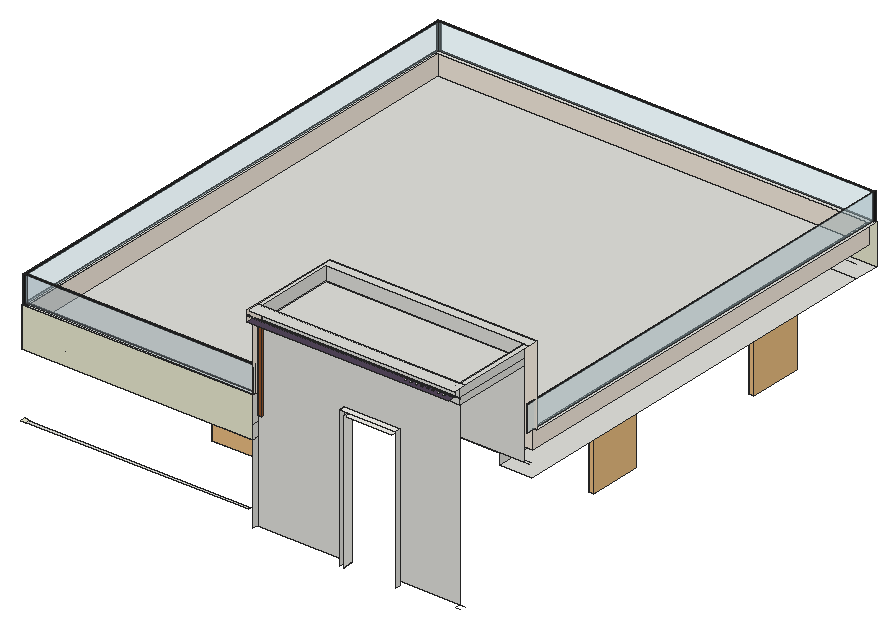
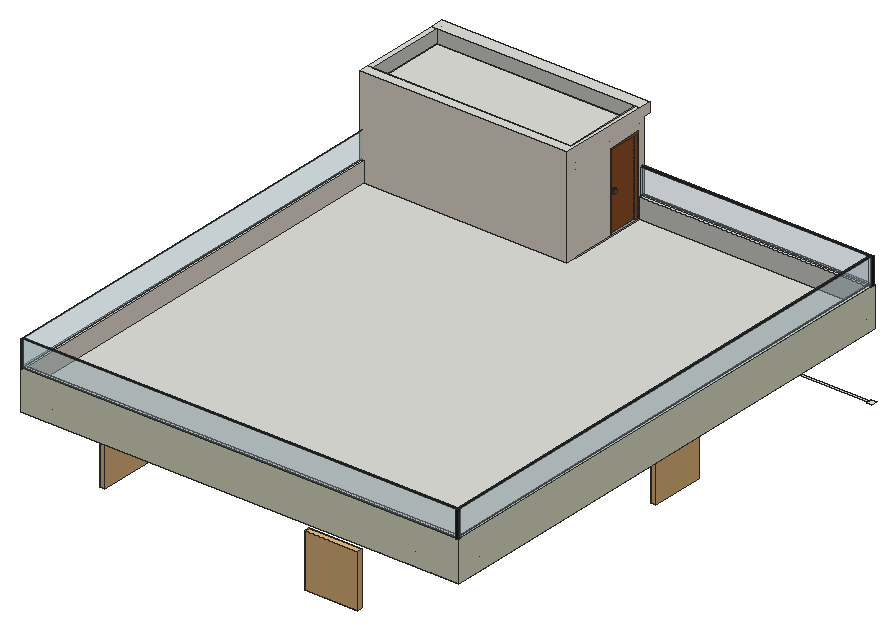
# SketchUp Ruby script. Lengths in inches.
U = 1.inch
M = Sketchup.active_model
def pt(a) = Geom::Point3d.new(a.map { |v| v * U })
def face(e, loops, mat)
  f = e.add_face(loops[0].map { |a| pt(a) })
  loops[1..].each { |l| e.add_face(l.map { |a| pt(a) }).erase! }
  f.material = f.back_material = mat if mat
  f
end
# faces: each face lists its corners as indices into pts; further lists are holes
def faces(e, pts, list, mat = nil) = list.each { |f| face(e, (f[0].is_a?(Array) ? f : [f]).map { |l| l.map { |i| pts[i] } }, mat) }
# xy, xz, yz: faces in a plane at the given z, y or x. An outline is a flat list of corners, or four numbers for a rectangle; further outlines are holes
def ring(l) = l.size == 4 ? [[l[0], l[1]], [l[2], l[1]], [l[2], l[3]], [l[0], l[3]]] : l.each_slice(2).to_a
def flat(e, list, mat, &to3) = list.each { |f| face(e, (f[0].is_a?(Array) ? f : [f]).map { |l| ring(l).map { |u, v| to3.(u, v) } }, mat) }
def xy(e, z, list, mat = nil) = flat(e, list, mat) { |x, y| [x, y, z] }
def xz(e, y, list, mat = nil) = flat(e, list, mat) { |x, z| [x, y, z] }
def yz(e, x, list, mat = nil) = flat(e, list, mat) { |y, z| [x, y, z] }
def lines(e, pts, list) = list.each { |a, b| e.add_line(pt(pts[a]), pt(pts[b])) }
# prism: a flat outline (further loops are holes) pulled along v
def prism(e, loops, v, mat = nil)
  f = face(e, loops, mat); d = Geom::Vector3d.new(v.map { |x| x * U })
  f.pushpull(f.normal.samedirection?(d) ? d.length : -d.length)
end
def box(e, o, s, mat = nil) = prism(e, [[o, [o[0] + s[0], o[1], o[2]], [o[0] + s[0], o[1] + s[1], o[2]], [o[0], o[1] + s[1], o[2]]]], [0, 0, s[2]], mat)
def at(x, y, z, deg = 0) = Geom::Transformation.translation(pt([x, y, z])) * Geom::Transformation.rotation(ORIGIN, Z_AXIS, deg.degrees)
def axes(o, x, y, z) = Geom::Transformation.new([*x, 0, *y, 0, *z, 0, *pt(o).to_a, 1])
def part(name) = M.definitions.add(name)
# library, detail: a bought-in or finely detailed component or shape, given as its bounding box
def library(name, o, s) = part(name).tap { |d| box(d.entities, o, s) }
def detail(e, o, s) = box(e.add_group.entities, o, s)
def put(e, d, t, mat = nil) = e.add_instance(d, t).tap { |i| i.material = mat if mat }
def group(e, t, mat = nil) = e.add_group.tap { |g| g.transformation = t; g.material = mat if mat }.entities
root = M.entities
M.materials.add("0037 AP 8028 PEACH ORGANZA").color = [246, 236, 223]
M.materials.add("0113 AP L161 ABSOLUTE WHITE").color = [243, 242, 236]
M.materials.add("0280 AP 9627 Emperor_s Purple-N").color = [83, 70, 91]
M.materials.add("0746 AP 7715 LUMINOUS").color = [235, 235, 209]
M.materials.add("Glass_Basic_01").color = [161, 173, 186]
M.materials["Glass_Basic_01"].alpha = 0.25
M.materials.add("Glass_Safety_01").color = [204, 235, 244]
M.materials["Glass_Safety_01"].alpha = 0.25
M.materials.add("M08_Obsidian_Black").color = [30, 30, 30]
M.materials.add("[Color M00]").color = [255, 255, 255]
M.materials.add("[Color M08]").color = [30, 30, 30]
M.materials.add("[Wood_Cherry_Original]").color = [152, 86, 42]
M.materials.add("[Wood_Lumber_ButtJoined]").color = [164, 152, 112]
c1 = library("Slide Window 5'",[0,-2.02,0],[60,2.02,54])
c2 = part("Electrical junction box")
xy(c2.entities,0,[[0.77,1.5,0.75,1.502,0.64,1.512,0.518,1.557,0.411,1.632,0.328,1.733,0.273,1.851,0.25,1.98,0.262,2.11,0.307,2.232,0.382,2.339,0.483,2.422,0.601,2.477,0.73,2.5,0.75,2.498,0.86,2.488,0.982,2.443,1.089,2.368,1.172,2.267,1.227,2.149,1.25,2.02,1.238,1.89,1.193,1.768,1.118,1.661,1.017,1.578,0.899,1.523]],"[Color M00]")
xy(c2.entities,0,[[[0,0,1.5,4],[0.77,1.5,0.899,1.523,1.017,1.578,1.118,1.661,1.193,1.768,1.238,1.89,1.25,2.02,1.227,2.149,1.172,2.267,1.089,2.368,0.982,2.443,0.86,2.488,0.75,2.498,0.73,2.5,0.601,2.477,0.483,2.422,0.382,2.339,0.307,2.232,0.262,2.11,0.25,1.98,0.273,1.851,0.328,1.733,0.411,1.632,0.518,1.557,0.64,1.512,0.75,1.502]]],"[Color M08]")
xy(c2.entities,4,[[0.75,1.502,0.879,1.525,0.997,1.579,1.097,1.663,1.172,1.77,1.217,1.892,1.229,2.022,1.207,2.151,1.152,2.269,1.068,2.37,0.962,2.445,0.839,2.49,0.75,2.498,0.73,2.5,0.709,2.501,0.581,2.479,0.462,2.424,0.362,2.341,0.287,2.234,0.242,2.111,0.23,1.981,0.252,1.853,0.307,1.734,0.391,1.634,0.497,1.559,0.62,1.514,0.73,1.504]],"[Color M00]")
xy(c2.entities,4,[[[0,0,1.5,4],[0.75,1.502,0.73,1.504,0.62,1.514,0.497,1.559,0.391,1.634,0.307,1.734,0.252,1.853,0.23,1.981,0.242,2.111,0.287,2.234,0.362,2.341,0.462,2.424,0.581,2.479,0.709,2.501,0.73,2.5,0.75,2.498,0.839,2.49,0.962,2.445,1.068,2.37,1.152,2.269,1.207,2.151,1.229,2.022,1.217,1.892,1.172,1.77,1.097,1.663,0.997,1.579,0.879,1.525]]],"[Color M08]")
xz(c2.entities,0,[[0.77,1.5,0.899,1.523,1.017,1.578,1.118,1.661,1.193,1.768,1.238,1.89,1.25,2.02,1.227,2.149,1.172,2.267,1.089,2.368,0.982,2.443,0.86,2.488,0.75,2.498,0.73,2.5,0.601,2.477,0.483,2.422,0.382,2.339,0.307,2.232,0.262,2.11,0.25,1.98,0.273,1.851,0.328,1.733,0.411,1.632,0.518,1.557,0.64,1.512,0.75,1.502]],"[Color M00]")
xz(c2.entities,0,[[[0,0,1.5,4],[0.77,1.5,0.75,1.502,0.64,1.512,0.518,1.557,0.411,1.632,0.328,1.733,0.273,1.851,0.25,1.98,0.262,2.11,0.307,2.232,0.382,2.339,0.483,2.422,0.601,2.477,0.73,2.5,0.75,2.498,0.86,2.488,0.982,2.443,1.089,2.368,1.172,2.267,1.227,2.149,1.25,2.02,1.238,1.89,1.193,1.768,1.118,1.661,1.017,1.578,0.899,1.523]]],"[Color M08]")
xz(c2.entities,4,[[0.73,1.5,0.601,1.523,0.483,1.578,0.382,1.661,0.307,1.768,0.262,1.89,0.25,2.02,0.273,2.149,0.328,2.267,0.411,2.368,0.518,2.443,0.64,2.488,0.75,2.498,0.77,2.5,0.899,2.477,1.017,2.422,1.118,2.339,1.193,2.232,1.238,2.11,1.25,1.98,1.227,1.851,1.172,1.733,1.089,1.632,0.982,1.557,0.86,1.512,0.75,1.502]],"[Color M00]")
xz(c2.entities,4,[[[0,0,1.5,4],[0.73,1.5,0.75,1.502,0.86,1.512,0.982,1.557,1.089,1.632,1.172,1.733,1.227,1.851,1.25,1.98,1.238,2.11,1.193,2.232,1.118,2.339,1.017,2.422,0.899,2.477,0.77,2.5,0.75,2.498,0.64,2.488,0.518,2.443,0.411,2.368,0.328,2.267,0.273,2.149,0.25,2.02,0.262,1.89,0.307,1.768,0.382,1.661,0.483,1.578,0.601,1.523]]],"[Color M08]")
yz(c2.entities,0,[[0,0,4,4]],"[Color M08]")
yz(c2.entities,1.5,[[0,0,4,4]],"[Color M08]")
p = [[0.75,2.498,4],[0.75,2.502,4]]
lines(c2.entities,p,[[0,1]])
c3 = library("Group\#25",[0,-0.05,0],[30,2.55,24])
xy(root,164.58,[[2160.9,113.67,2361.69,115.67]])
xy(root,164.58,[[2155.9,112.36,2160.9,117.37]],"0746 AP 7715 LUMINOUS")
xy(root,199.5,[[2205.9,189.89,2253.93,198.88],[2427.9,198.88,2432.9,228.89],[2196.91,383.38,2205.9,431.37],[2427.9,383.38,2432.9,413.39]])
xy(root,223.5,[[2157.2,112.36,2196.91,121.52],[2196.91,112.36,2366.69,121.52],[2157.2,121.52,2196.91,560.39],[2525.88,192.78,2554.91,560.39],[2157.2,560.39,2196.91,583.09],
  [2196.91,560.39,2525.88,583.09],[2525.88,560.39,2554.91,583.09]])
xy(root,235.5,[[[2196.91,121.52,2366.69,121.52,2366.69,189.89,2525.88,189.89,2525.88,560.39,2196.91,560.39,2196.91,431.37,2205.9,431.37,2205.9,383.38,2196.91,383.38],[2205.9,189.89,2253.93,198.88],[2427.9,383.38,2432.9,413.39],[2427.9,198.88,2432.9,228.89]],[2205.9,189.89,2253.93,198.88],[2427.9,198.88,2432.9,228.89],[2196.91,383.38,2205.9,431.37],[2427.9,383.38,2432.9,413.39]])
xy(root,240,[[2196.98,190.05,2525.95,560.55]])
xy(root,241.5,[[2161.2,117.37,2366.69,117.37,2366.69,198.89,2550.91,198.89,2550.91,579.09,2161.2,579.09],[2369.92,118.67,2371.21,149.31],[2366.69,150.93,2370.69,189.89]])
xy(root,241.5,[[2366.93,117.05,2366.93,119.07,2369.92,119.07,2369.92,118.67,2371.21,118.67,2371.21,117.05],[2366.93,148.91,2366.93,150.93,2371.21,150.93,2371.21,149.31,2369.92,149.31,2369.92,148.91]],"[Wood_Cherry_Original]")
xy(root,259.5,[[2157.2,112.36,2161.2,579.09],[2161.2,112.36,2366.69,117.37],[2550.91,198.89,2554.91,583.09],[2157.2,579.09,2550.91,583.09]])
xy(root,274.5,[[2452.6,108.36,2495.6,117.37]],"0113 AP L161 ABSOLUTE WHITE")
xy(root,275.5,[[2366.93,144.21,2369.92,146.17]],"[Wood_Cherry_Original]")
xy(root,276.69,[[2368.32,142.55,2368.45,142.75]],"[Wood_Lumber_ButtJoined]")
xy(root,278.26,[[2366.93,144.21,2369.92,146.17]],"[Wood_Cherry_Original]")
xy(root,278.5,[[2448.6,108.36,2499.54,112.36]],"0113 AP L161 ABSOLUTE WHITE")
xy(root,311.42,[[2366.93,119.07,2369.92,148.91]],"[Wood_Cherry_Original]")
xy(root,311.78,[[2369.92,118.67,2371.21,149.31]])
xy(root,313.5,[[2371.21,117.37,2371.21,150.93,2370.69,150.93,2370.69,189.89,2549.9,189.89,2549.9,117.37]])
xy(root,313.5,[[2366.93,117.05,2371.21,117.37],[2366.93,117.37,2370.69,150.93],[2370.69,117.37,2371.21,150.93]],"[Wood_Cherry_Original]")
xy(root,319.5,[[2370.69,117.37,2549.9,189.89]])
xy(root,322.5,[[2506.22,109.7,2507.72,110.7],[2511.22,109.7,2512.72,110.7],[2516.22,109.7,2517.72,110.7],[2521.22,109.7,2522.72,110.7],[2526.22,109.7,2527.72,110.7],
  [2531.22,109.7,2532.72,110.7],[2536.22,109.7,2537.72,110.7],[2541.22,109.7,2542.72,110.7]])
xy(root,322.5,[[[2366.69,105.36,2549.9,112.36],[2506.22,109.7,2507.72,110.7],[2511.22,109.7,2512.72,110.7],[2516.22,109.7,2517.72,110.7],[2521.22,109.7,2522.72,110.7],[2526.22,109.7,2527.72,110.7],[2531.22,109.7,2532.72,110.7],[2536.22,109.7,2537.72,110.7],[2541.22,109.7,2542.72,110.7]]],"0280 AP 9627 Emperor_s Purple-N")
xy(root,327,[[2366.69,105.16,2552.4,105.36]])
xy(root,327.8,[[2366.69,105.16,2553.2,105.36]])
xy(root,331.5,[[2366.69,105.36,2554.91,117.37],[2366.69,117.37,2370.69,117.37,2370.69,189.89,2554.91,189.89,2554.91,198.89,2366.69,198.89],[2549.9,117.37,2554.91,189.89]])
xz(root,112.36,[[2157.2,223.5,2366.69,259.5]],"0746 AP 7715 LUMINOUS")
xz(root,117.05,[[2366.93,241.5,2371.21,313.5]],"[Wood_Cherry_Original]")
xz(root,117.37,[[2366.69,151.5,2366.69,313.5,2549.9,313.5,2549.9,151.5,2495.6,151.5,2495.6,274.5,2452.6,274.5,2452.6,151.5],[2161.2,241.5,2366.69,259.5],[2370.69,313.5,2549.9,319.5],[2370.69,319.5,2549.9,331.5]])
xz(root,118.67,[[2369.92,241.5,2371.21,311.78]])
xz(root,119.07,[[2366.93,241.5,2369.92,311.42]],"[Wood_Cherry_Original]")
xz(root,121.52,[[2196.91,223.5,2366.69,235.5]])
xz(root,142.55,[[[2368.42,276.35,2368.28,276.37,2368.15,276.42,2368.04,276.5,2367.96,276.61,2367.9,276.74,2367.88,276.87,2367.9,277.01,2367.96,277.13,2368.04,277.24,2368.15,277.32,2368.28,277.375,2368.42,277.39,2368.56,277.375,2368.6875,277.32,2368.8,277.24,2368.88,277.13,2368.9375,277.01,2368.96,276.87,2368.9375,276.74,2368.88,276.61,2368.8,276.5,2368.6875,276.42,2368.56,276.37],[2368.32,276.69,2368.45,276.69,2368.45,276.9,2368.49,276.94,2368.5,276.96,2368.51,276.99,2368.5,277.02,2368.49,277.04,2368.47,277.07,2368.43,277.09,2368.4,277.1,2368.34,277.08,2368.32,277.07,2368.31,277.04,2368.29,277.02,2368.29,276.96,2368.31,276.94,2368.32,276.92]]],"[Wood_Cherry_Original]")
xz(root,142.75,[[2368.32,276.69,2368.32,276.92,2368.34,276.9,2368.37,276.89,2368.43,276.89,2368.45,276.9,2368.45,276.69],[2368.37,276.89,2368.34,276.9,2368.32,276.92,2368.31,276.94,2368.29,276.96,2368.29,277.02,2368.31,277.04,2368.32,277.07,2368.34,277.08,2368.4,277.1,2368.43,277.09,2368.47,277.07,2368.49,277.04,2368.5,277.02,2368.51,276.99,2368.5,276.96,2368.49,276.94,2368.45,276.9,2368.43,276.89]],"[Wood_Lumber_ButtJoined]")
xz(root,144.21,[[[2366.93,275.5,2369.92,278.26],[2368.42,276.35,2368.56,276.37,2368.6875,276.42,2368.8,276.5,2368.88,276.61,2368.9375,276.74,2368.96,276.87,2368.9375,277.01,2368.88,277.13,2368.8,277.24,2368.6875,277.32,2368.56,277.375,2368.42,277.39,2368.28,277.375,2368.15,277.32,2368.04,277.24,2367.96,277.13,2367.9,277.01,2367.88,276.87,2367.9,276.74,2367.96,276.61,2368.04,276.5,2368.15,276.42,2368.28,276.37]]],"[Wood_Cherry_Original]")
xz(root,146.17,[[2366.93,275.5,2369.92,278.26]],"[Wood_Cherry_Original]")
xz(root,148.91,[[2366.93,241.5,2369.92,311.42]],"[Wood_Cherry_Original]")
xz(root,149.31,[[2369.92,241.5,2371.21,311.78]])
xz(root,150.93,[[2366.93,241.5,2370.69,313.5]])
xz(root,150.93,[[2370.69,241.5,2371.21,313.5]],"[Wood_Cherry_Original]")
xz(root,189.89,[[2366.69,235.5,2549.9,235.5,2549.9,313.5,2370.69,313.5,2370.69,241.5,2366.69,241.5],[2370.69,313.5,2549.9,319.5],[2370.69,319.5,2549.9,331.5]])
xz(root,189.89,[[2205.9,199.5,2253.93,235.5]],"0037 AP 8028 PEACH ORGANZA")
xz(root,198.88,[[2205.9,199.5,2253.93,235.5],[2427.9,199.5,2432.9,235.5]])
xz(root,198.89,[[2366.69,241.5,2366.69,331.5,2554.91,331.5,2554.91,259.5,2550.91,259.5,2550.91,241.5]],"0037 AP 8028 PEACH ORGANZA")
xz(root,228.89,[[2427.9,199.5,2432.9,235.5]])
xz(root,383.38,[[2196.91,199.5,2205.9,235.5],[2427.9,199.5,2432.9,235.5]])
xz(root,413.39,[[2427.9,199.5,2432.9,235.5]])
xz(root,431.37,[[2196.91,199.5,2205.9,235.5]])
xz(root,560.39,[[2196.91,223.5,2525.88,235.5]])
xz(root,579.09,[[2161.2,241.5,2550.91,259.5]],"0037 AP 8028 PEACH ORGANZA")
xz(root,583.09,[[2157.2,223.5,2554.91,259.5]],"0746 AP 7715 LUMINOUS")
yz(root,2157.2,[[112.36,223.5,583.09,259.5]],"0746 AP 7715 LUMINOUS")
yz(root,2161.2,[[117.37,241.5,579.09,259.5]],"0037 AP 8028 PEACH ORGANZA")
yz(root,2196.91,[[121.52,223.5,383.38,235.5],[383.38,223.5,431.37,235.5],[431.37,223.5,560.39,235.5]])
yz(root,2196.91,[[383.38,199.5,431.37,223.5]],"0037 AP 8028 PEACH ORGANZA")
yz(root,2205.9,[[189.89,199.5,198.88,235.5],[383.38,199.5,431.37,235.5]])
yz(root,2253.93,[[189.89,199.5,198.88,235.5]])
yz(root,2365.27,[[[146.17,275.5,146.51,275.54,146.84,275.68,147.11,275.9,147.33,276.1875,147.46,276.52,147.5,276.875,147.46,277.23,147.33,277.57,147.11,277.85,146.84,278.07,146.51,278.21,146.17,278.26,145.82,278.21,145.5,278.07,145.22,277.85,145.01,277.57,144.88,277.23,144.83,276.875,144.88,276.52,145.01,276.1875,145.22,275.9,145.5,275.68,145.82,275.54],[146.2,276.36,146.07,276.375,145.95,276.43,145.84,276.51,145.76,276.62,145.71,276.74,145.7,276.88,145.71,277.01,145.76,277.14,145.84,277.25,145.95,277.33,146.07,277.38,146.2,277.4,146.33,277.38,146.45,277.33,146.56,277.25,146.64,277.14,146.6875,277.01,146.7,276.88,146.6875,276.74,146.64,276.62,146.56,276.51,146.45,276.43,146.33,276.375]]],"[Wood_Cherry_Original]")
yz(root,2365.91,[[146.2,276.36,146.33,276.375,146.45,276.43,146.56,276.51,146.64,276.62,146.6875,276.74,146.7,276.88,146.6875,277.01,146.64,277.14,146.56,277.25,146.45,277.33,146.33,277.38,146.2,277.4,146.07,277.38,145.95,277.33,145.84,277.25,145.76,277.14,145.71,277.01,145.7,276.88,145.71,276.74,145.76,276.62,145.84,276.51,145.95,276.43,146.07,276.375]],"[Wood_Cherry_Original]")
yz(root,2366.69,[[112.36,151.5,117.37,223.5],[112.36,223.5,117.37,235.5],[117.37,223.5,121.52,235.5],[112.36,235.5,117.37,259.5],[117.37,235.5,189.89,241.5]])
yz(root,2366.69,[[150.93,241.5,150.93,313.5,117.37,313.5,117.37,259.5,112.36,259.5,112.36,322.5,105.36,322.5,105.36,327,105.16,327,105.16,327.8,105.36,327.8,105.36,331.5,198.89,331.5,198.89,241.5]],"0037 AP 8028 PEACH ORGANZA")
yz(root,2366.93,[[146.17,275.5,146.51,275.54,146.84,275.68,147.11,275.9,147.33,276.1875,147.46,276.52,147.5,276.875,147.46,277.23,147.33,277.57,147.11,277.85,146.84,278.07,146.51,278.21,146.17,278.26]])
yz(root,2366.93,[[117.05,241.5,117.05,313.5,119.07,311.42,119.07,241.5],[148.91,241.5,148.91,311.42,150.93,313.5,150.93,241.5],[144.21,275.5,146.17,275.5,145.82,275.54,145.5,275.68,145.22,275.9,145.01,276.1875,144.88,276.52,144.83,276.875,144.88,277.23,145.01,277.57,145.22,277.85,145.5,278.07,145.82,278.21,146.17,278.26,144.21,278.26],[119.07,311.42,117.05,313.5,150.93,313.5,148.91,311.42]],"[Wood_Cherry_Original]")
yz(root,2368.29,[[142.55,276.96,142.75,276.99],[142.55,276.99,142.75,277.02]],"[Wood_Lumber_ButtJoined]")
yz(root,2368.32,[[142.55,276.69,142.75,276.92]],"[Wood_Lumber_ButtJoined]")
yz(root,2368.45,[[142.55,276.69,142.75,276.9]],"[Wood_Lumber_ButtJoined]")
yz(root,2369.92,[[118.67,241.5,119.07,241.5,119.07,311.42,148.91,311.42,148.91,241.5,149.31,241.5,149.31,311.78,118.67,311.78]])
yz(root,2369.92,[[[119.07,241.5,148.91,311.42],[144.21,275.5,146.17,278.26]]],"[Wood_Cherry_Original]")
yz(root,2370.69,[[150.93,241.5,189.89,313.5],[117.37,313.5,150.93,319.5],[150.93,313.5,189.89,319.5],[117.37,319.5,189.89,331.5]])
yz(root,2371.21,[[117.05,241.5,118.67,313.5],[118.67,241.5,149.31,311.78],[149.31,241.5,150.93,313.5],[118.67,311.78,149.31,313.5]],"[Wood_Cherry_Original]")
yz(root,2427.9,[[198.88,199.5,228.89,235.5],[383.38,199.5,413.39,235.5]])
yz(root,2432.9,[[198.88,199.5,228.89,235.5],[383.38,199.5,413.39,235.5]])
yz(root,2448.6,[[108.36,151.5,112.36,278.5]])
yz(root,2452.6,[[108.36,151.49,117.37,151.5]])
yz(root,2452.6,[[108.36,151.5,117.37,274.5]],"0113 AP L161 ABSOLUTE WHITE")
yz(root,2499.54,[[108.36,151.5,112.36,278.5]])
yz(root,2525.88,[[192.78,223.5,560.39,235.5]])
yz(root,2549.9,[[117.37,313.5,189.89,319.5],[117.37,319.5,189.89,331.5]])
yz(root,2550.91,[[198.89,241.5,579.09,259.5]],"0037 AP 8028 PEACH ORGANZA")
yz(root,2553.2,[[105.16,327,105.36,327.8]])
p = [[2366.93,145.5,275.68],[2366.93,145.82,275.54],[2365.27,145.82,275.54],[2365.27,145.5,275.68],[2366.93,146.17,275.5],[2365.27,146.17,275.5],
  [2366.93,146.51,275.54],[2365.27,146.51,275.54],[2366.93,146.84,275.68],[2365.27,146.84,275.68],[2366.93,145.22,275.9],[2365.27,145.22,275.9],
  [2366.93,147.11,275.9],[2365.27,147.11,275.9],[2366.93,145.01,276.1875],[2365.27,145.01,276.1875],[2366.93,147.33,276.1875],[2365.27,147.33,276.1875],
  [2366.93,144.88,276.52],[2365.27,144.88,276.52],[2366.93,147.46,276.52],[2365.27,147.46,276.52],[2368.15,144.21,276.42],[2368.04,144.21,276.5],
  [2368.04,142.55,276.5],[2368.15,142.55,276.42],[2368.28,144.21,276.37],[2368.28,142.55,276.37],[2368.42,144.21,276.35],[2368.42,142.55,276.35],
  [2368.56,144.21,276.37],[2368.56,142.55,276.37],[2368.6875,144.21,276.42],[2368.6875,142.55,276.42],[2368.8,144.21,276.5],[2368.8,142.55,276.5],
  [2365.27,145.84,276.51],[2365.27,145.95,276.43],[2365.91,145.95,276.43],[2365.91,145.84,276.51],[2365.27,146.07,276.375],[2365.91,146.07,276.375],
  [2365.27,146.2,276.36],[2365.91,146.2,276.36],[2365.27,146.33,276.375],[2365.91,146.33,276.375],[2365.27,146.45,276.43],[2365.91,146.45,276.43],
  [2365.27,146.56,276.51],[2365.91,146.56,276.51],[2367.96,144.21,276.61],[2367.96,142.55,276.61],[2368.88,144.21,276.61],[2368.88,142.55,276.61],
  [2366.93,144.83,276.875],[2365.27,144.83,276.875],[2365.27,145.76,276.62],[2365.91,145.76,276.62],[2365.27,146.64,276.62],[2365.91,146.64,276.62],
  [2366.93,147.5,276.875],[2365.27,147.5,276.875],[2367.9,144.21,276.74],[2367.9,142.55,276.74],[2368.9375,144.21,276.74],[2368.9375,142.55,276.74],
  [2365.27,145.71,276.74],[2365.91,145.71,276.74],[2365.27,146.6875,276.74],[2365.91,146.6875,276.74],[2367.88,144.21,276.87],[2367.88,142.55,276.87],
  [2368.96,144.21,276.87],[2368.96,142.55,276.87],[2365.27,145.7,276.88],[2365.91,145.7,276.88],[2365.27,146.7,276.88],[2365.91,146.7,276.88],
  [2367.9,144.21,277.01],[2367.9,142.55,277.01],[2368.32,142.55,276.92],[2368.31,142.55,276.94],[2368.31,142.75,276.94],[2368.32,142.75,276.92],
  [2368.29,142.55,276.96],[2368.29,142.75,276.96],[2368.47,142.55,276.92],[2368.45,142.55,276.9],[2368.45,142.75,276.9],[2368.47,142.75,276.92],
  [2368.49,142.55,276.94],[2368.49,142.75,276.94],[2368.5,142.55,276.96],[2368.5,142.75,276.96],[2368.9375,144.21,277.01],[2368.9375,142.55,277.01],
  [2366.93,144.88,277.23],[2365.27,144.88,277.23],[2365.27,145.71,277.01],[2365.91,145.71,277.01],[2365.27,146.6875,277.01],[2365.91,146.6875,277.01],
  [2366.93,147.46,277.23],[2365.27,147.46,277.23],[2367.96,144.21,277.13],[2367.96,142.55,277.13],[2368.29,142.55,277.02],[2368.31,142.55,277.04],
  [2368.31,142.75,277.04],[2368.29,142.75,277.02],[2368.32,142.55,277.07],[2368.32,142.75,277.07],[2368.51,142.55,276.99],[2368.51,142.75,276.99],
  [2368.5,142.55,277.02],[2368.5,142.75,277.02],[2368.49,142.55,277.04],[2368.49,142.75,277.04],[2368.47,142.55,277.07],[2368.47,142.75,277.07],
  [2368.88,144.21,277.13],[2368.88,142.55,277.13],[2365.27,145.76,277.14],[2365.91,145.76,277.14],[2365.27,146.64,277.14],[2365.91,146.64,277.14],
  [2368.04,144.21,277.24],[2368.04,142.55,277.24],[2368.34,142.55,277.08],[2368.34,142.75,277.08],[2368.37,142.55,277.09],[2368.37,142.75,277.09],
  [2368.43,142.55,277.09],[2368.45,142.55,277.08],[2368.45,142.75,277.08],[2368.43,142.75,277.09],[2368.4,142.55,277.1],[2368.4,142.75,277.1],
  [2368.8,144.21,277.24],[2368.8,142.55,277.24],[2365.27,145.84,277.25],[2365.91,145.84,277.25],[2365.27,146.56,277.25],[2365.91,146.56,277.25],
  [2368.15,144.21,277.32],[2368.15,142.55,277.32],[2368.6875,144.21,277.32],[2368.6875,142.55,277.32],[2366.93,145.01,277.57],[2365.27,145.01,277.57],
  [2365.27,145.95,277.33],[2365.91,145.95,277.33],[2365.27,146.45,277.33],[2365.91,146.45,277.33],[2366.93,147.33,277.57],[2365.27,147.33,277.57],
  [2368.28,144.21,277.375],[2368.28,142.55,277.375],[2368.56,144.21,277.375],[2368.56,142.55,277.375],[2365.27,146.07,277.38],[2365.91,146.07,277.38],
  [2365.27,146.33,277.38],[2365.91,146.33,277.38],[2368.42,144.21,277.39],[2368.42,142.55,277.39],[2365.27,146.2,277.4],[2365.91,146.2,277.4],
  [2366.93,145.22,277.85],[2365.27,145.22,277.85],[2366.93,147.11,277.85],[2365.27,147.11,277.85],[2366.93,145.5,278.07],[2365.27,145.5,278.07],
  [2366.93,146.84,278.07],[2365.27,146.84,278.07],[2366.93,145.82,278.21],[2365.27,145.82,278.21],[2366.93,146.51,278.21],[2365.27,146.51,278.21],
  [2366.93,146.17,278.26],[2365.27,146.17,278.26],[2370.76,117.27,240.79],[2370.76,149.89,240.66],[2554.91,189.89,235.5],[2549.9,189.89,235.5],
  [2370.69,189.89,241.5],[2370.69,198.89,241.5],[2366.69,150.93,319.5],[2370.69,150.93,319.5],[2196.91,112.36,235.5],[2196.91,121.52,235.5],
  [2157.2,121.52,235.5],[2196.91,560.39,235.5],[2157.2,560.39,235.5],[2196.91,583.09,235.5],[2525.88,560.39,235.5],[2525.88,583.09,235.5],
  [2554.91,560.39,235.5],[2525.88,192.78,235.5],[2554.91,192.78,235.5],[2366.69,117.37,319.5],[2370.69,117.37,319.5],[2370.69,189.89,319.5],
  [2366.69,189.89,319.5],[2370.69,189.89,313.5],[2366.69,189.89,313.5],[2371.21,119.02,311.42],[2371.21,119.07,311.42],[2549.9,112.36,322.5],
  [2554.91,112.36,322.5],[2549.9,117.37,151.5],[2549.9,112.36,151.5],[2549.9,112.36,331.5],[2554.91,117.37,151.5],[2554.91,112.36,151.5]]
faces(root,p,[[0,1,2,3],[1,4,5,2],[6,4,5,7],[8,6,7,9],[10,0,3,11],[12,8,9,13],[14,10,11,15],[16,12,13,17],
  [18,14,15,19],[20,16,17,21],[22,23,24,25],[26,22,25,27],[28,26,27,29],[30,28,29,31],[32,30,31,33],[34,32,33,35],
  [36,37,38,39],[37,40,41,38],[40,42,43,41],[42,44,45,43],[44,46,47,45],[46,48,49,47],[23,50,51,24],[52,34,35,53],
  [54,18,19,55],[56,36,39,57],[48,58,59,49],[60,20,21,61],[50,62,63,51],[64,52,53,65],[66,56,57,67],[58,68,69,59],
  [62,70,71,63],[72,64,65,73],[74,66,67,75],[68,76,77,69],[70,78,79,71],[94,72,73,95],[96,54,55,97],[98,74,75,99],
  [76,100,101,77],[102,60,61,103],[78,104,105,79],[120,94,95,121],[122,98,99,123],[100,124,125,101],[104,126,127,105],[138,120,121,139],
  [140,122,123,141],[124,142,143,125],[126,144,145,127],[146,138,139,147],[148,96,97,149],[150,140,141,151],[142,152,153,143],[154,102,103,155],
  [144,156,157,145],[158,146,147,159],[160,150,151,161],[152,162,163,153],[156,164,165,157],[164,158,159,165],[166,160,161,167],[162,166,167,163],
  [168,148,149,169],[170,154,155,171],[172,168,169,173],[174,170,171,175],[176,172,173,177],[178,174,175,179],[180,176,177,181],[180,178,179,181]],"[Wood_Cherry_Original]")
faces(root,p,[[80,81,82,83],[81,84,85,82],[86,87,88,89],[90,86,89,91],[92,90,91,93],[106,107,108,109],[107,110,111,108],[112,92,93,113],
  [114,112,113,115],[116,114,115,117],[118,116,117,119],[110,128,129,111],[128,130,131,129],[132,133,134,135],[136,132,135,137],[130,136,137,131],
  [133,118,119,134]],"[Wood_Lumber_ButtJoined]")
lines(root,p,[[182,183],[184,185],[186,187],[188,189],[190,191],[191,192],[193,194],[193,195],[196,197],[196,198],[199,200],[201,202],
  [203,204],[205,206],[207,208],[209,210],[211,212],[209,213],[211,214],[212,215]])
put(root,c1,axes([2523.53,531.92,151.02],[0,-0.8005,0],[2.31,0,0],[0,0,0.89771]))
put(root,c1,axes([2523.37,350.42,151.44],[0,-0.80083,0],[2.31,0,0],[0,0,0.89771]))
put(root,c1,axes([2268.87,558.14,151.5],[0.79979,0,0],[0,2.31,0],[0,0,0.88889]))
put(root,c1,axes([2198.76,260.14,151.82],[0,0.79979,0],[-2.31,0,0],[0,0,1.3273]))
put(root,c1,axes([2265.93,196.46,152.5],[0.8,0,0],[0,2.31,0],[0,0,0.88889]))
put(root,c2,axes([2330.2,189.89,169.87],[0,-3.6442,0],[0.70711,0,-0.70711],[0.70711,0,0.70711]))
put(root,c3,axes([2518.89,231.88,211.42],[0,-0.60073,0],[1.82683,0,0],[0,0,0.50315]))
put(root,c3,axes([2518.89,417.37,211.42],[0,-0.66205,0],[1.82683,0,0],[0,0,0.51171]))
g1 = group(root,at(2159.63,113.83,259.5),"Glass_Safety_01")
xy(g1,0,[[-2.52,0,0,2.02],[0,0,207.0625,2.02],[-2.52,2.02,0,468.3],[392.68,76.12,393.6875,468.3],[-2.52,468.3,0,470.16],
  [0,468.3,392.68,470.16],[392.68,468.3,393.6875,470.16]])
xy(g1,24,[[-2.52,0,0,2.02],[0,0,207.0625,2.02],[-2.52,2.02,0,468.3],[392.68,76.12,393.6875,468.3],[-2.52,468.3,0,470.16],
  [0,468.3,392.68,470.16],[392.68,468.3,393.6875,470.16]],"M08_Obsidian_Black")
xz(g1,0,[[0,0,207.0625,24]],"Glass_Basic_01")
xz(g1,0,[[-2.52,0,0,24]],"M08_Obsidian_Black")
xz(g1,2.02,[[-2.52,0,0,24],[0,0,207.0625,24]])
xz(g1,76.12,[[392.68,0,393.6875,24]])
xz(g1,468.3,[[-2.52,0,0,24],[0,0,392.68,24],[392.68,0,393.6875,24]])
xz(g1,470.16,[[0,0,392.68,24]])
xz(g1,470.16,[[-2.52,0,0,24],[392.68,0,393.6875,24]],"M08_Obsidian_Black")
yz(g1,-2.52,[[2.02,0,468.3,24]])
yz(g1,-2.52,[[0,0,2.02,24],[468.3,0,470.16,24]],"M08_Obsidian_Black")
yz(g1,0,[[0,0,2.02,24],[2.02,0,468.3,24],[468.3,0,470.16,24]])
yz(g1,207.0625,[[0,0,2.02,24]])
yz(g1,392.68,[[76.12,0,468.3,24],[468.3,0,470.16,24]])
yz(g1,393.6875,[[76.12,0,468.3,24]])
yz(g1,393.6875,[[468.3,0,470.16,24]],"M08_Obsidian_Black")
